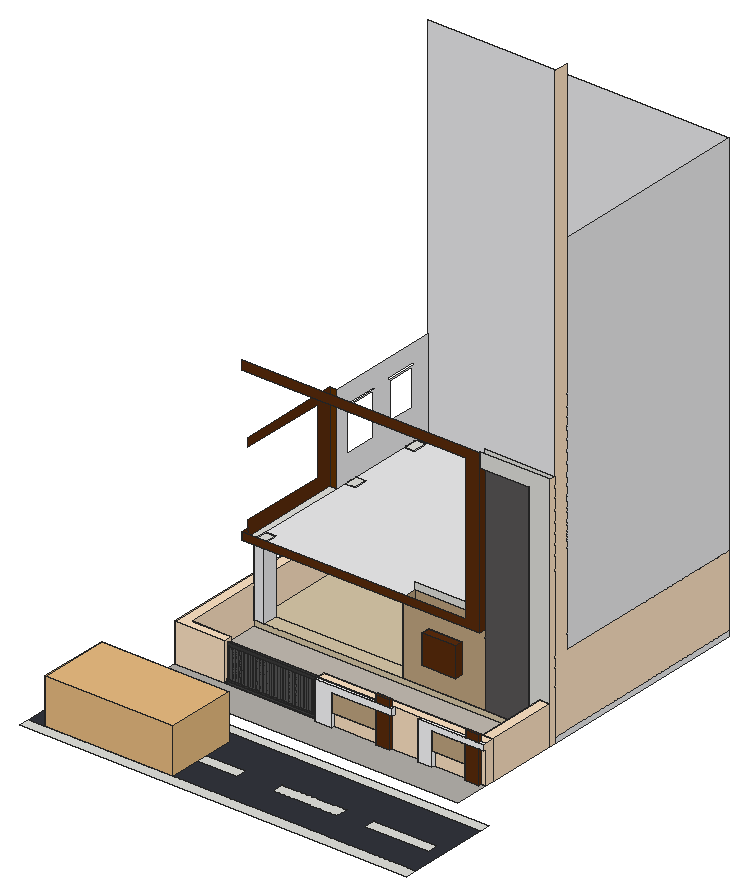
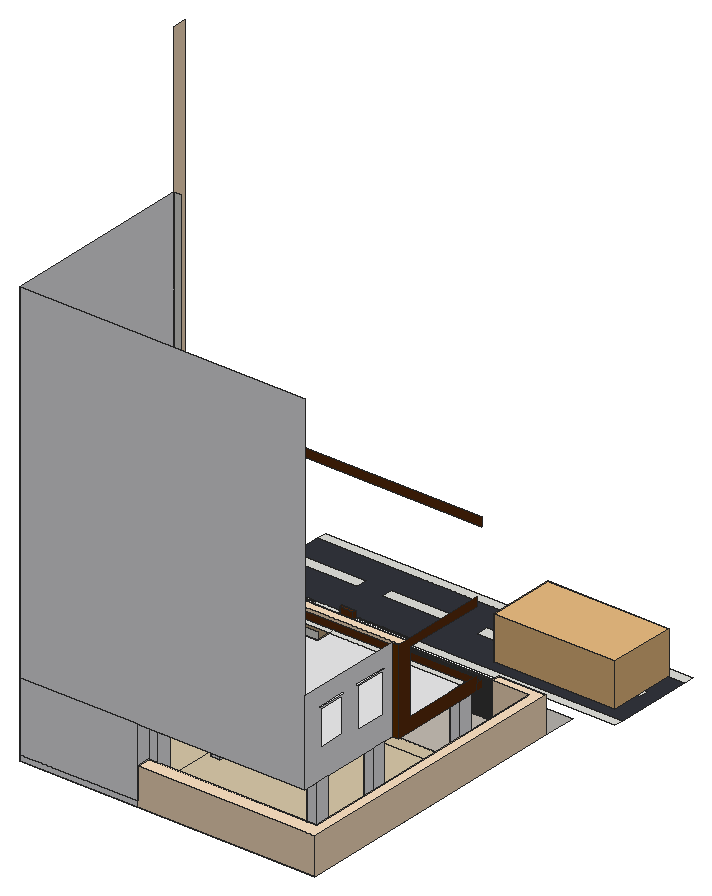
# SketchUp Ruby script. Lengths in inches.
U = 1.inch
M = Sketchup.active_model
def pt(a) = Geom::Point3d.new(a.map { |v| v * U })
def face(e, loops, mat)
  f = e.add_face(loops[0].map { |a| pt(a) })
  loops[1..].each { |l| e.add_face(l.map { |a| pt(a) }).erase! }
  f.material = f.back_material = mat if mat
  f
end
# faces: each face lists its corners as indices into pts; further lists are holes
def faces(e, pts, list, mat = nil) = list.each { |f| face(e, (f[0].is_a?(Array) ? f : [f]).map { |l| l.map { |i| pts[i] } }, mat) }
# xy, xz, yz: faces in a plane at the given z, y or x. An outline is a flat list of corners, or four numbers for a rectangle; further outlines are holes
def ring(l) = l.size == 4 ? [[l[0], l[1]], [l[2], l[1]], [l[2], l[3]], [l[0], l[3]]] : l.each_slice(2).to_a
def flat(e, list, mat, &to3) = list.each { |f| face(e, (f[0].is_a?(Array) ? f : [f]).map { |l| ring(l).map { |u, v| to3.(u, v) } }, mat) }
def xy(e, z, list, mat = nil) = flat(e, list, mat) { |x, y| [x, y, z] }
def xz(e, y, list, mat = nil) = flat(e, list, mat) { |x, z| [x, y, z] }
def yz(e, x, list, mat = nil) = flat(e, list, mat) { |y, z| [x, y, z] }
def lines(e, pts, list) = list.each { |a, b| e.add_line(pt(pts[a]), pt(pts[b])) }
# prism: a flat outline (further loops are holes) pulled along v
def prism(e, loops, v, mat = nil)
  f = face(e, loops, mat); d = Geom::Vector3d.new(v.map { |x| x * U })
  f.pushpull(f.normal.samedirection?(d) ? d.length : -d.length)
end
def box(e, o, s, mat = nil) = prism(e, [[o, [o[0] + s[0], o[1], o[2]], [o[0] + s[0], o[1] + s[1], o[2]], [o[0], o[1] + s[1], o[2]]]], [0, 0, s[2]], mat)
def at(x, y, z, deg = 0) = Geom::Transformation.translation(pt([x, y, z])) * Geom::Transformation.rotation(ORIGIN, Z_AXIS, deg.degrees)
def axes(o, x, y, z) = Geom::Transformation.new([*x, 0, *y, 0, *z, 0, *pt(o).to_a, 1])
def part(name) = M.definitions.add(name)
# library, detail: a bought-in or finely detailed component or shape, given as its bounding box
def library(name, o, s) = part(name).tap { |d| box(d.entities, o, s) }
def detail(e, o, s) = box(e.add_group.entities, o, s)
def put(e, d, t, mat = nil) = e.add_instance(d, t).tap { |i| i.material = mat if mat }
def group(e, t, mat = nil) = e.add_group.tap { |g| g.transformation = t; g.material = mat if mat }.entities
root = M.entities
M.materials.add("[0012_Bisque]").color = [255, 228, 196]
M.materials.add("[0035_Tan]").color = [188, 161, 125]
M.materials.add("[0035_Tan]1").color = [193, 166, 129]
M.materials.add("[0043_SaddleBrown]").color = [91, 44, 12]
M.materials.add("[Blinds Vertical Pattern]").color = [237, 237, 239]
M.materials.add("[Brick Tumbled]").color = [89, 87, 87]
M.materials.add("[Color C08]").color = [102, 51, 0]
M.materials.add("[Color M06]").color = [86, 86, 86]
M.materials.add("[Color M07]").color = [58, 58, 58]
M.materials.add("[Field Rectangle Tile]").color = [196, 189, 179]
M.materials.add("[Field Square Tile]").color = [217, 201, 169]
M.materials.add("[Formica Laminate Dark]1").color = [50, 53, 60]
M.materials.add("[Quartz Light Grey]").color = [251, 251, 252]
M.materials.add("[Tile Travertine 2 inch]").color = [181, 178, 172]
c1 = library("skpE847",[-111.76,-15.01,0.76],[2.12,4.6,1.82])
c2 = part("car+1")
p = [[0,0,0],[1,0,0],[1,1,0]]
lines(c2.entities,p,[[0,1],[1,2],[2,0]])
put(c2.entities,c1,axes([-477.97,5140.8,-31.25],[0,46,0],[-46,0,0],[0,0,40.94]))
xy(root,0,[[0,0,641.75,17.59],[22.28,68.03,129.53,88.03],[198.41,68.03,305.66,88.03],[364.41,68.03,471.66,88.03],[516.03,68.03,623.28,88.03],
  [0,153.78,641.75,169.75],[537.68,383.84,572.32,393.34],[56.22,393.34,572.32,753.91]])
xy(root,0,[[73.92,264.9,73.92,393.34,537.68,393.34,537.68,383.84,555.09,383.84,555.09,264.9]],"[Field Rectangle Tile]")
xy(root,0,[[[0,17.59,641.75,153.78],[516.03,68.03,623.28,88.03],[364.41,68.03,471.66,88.03],[198.41,68.03,305.66,88.03],[22.28,68.03,129.53,88.03]]],"[Formica Laminate Dark]1")
xy(root,0,[[292.71,246.01,320.3125,250.82],[392.59,246.01,416.02,250.82],[463.56,246.01,486.63,250.82],[541.28,246.01,564.49,250.82],[56.22,250.82,56.22,393.34,73.92,393.34,73.92,264.9,138.4,264.9,138.4,250.82],
  [138.4,250.82,292.71,264.9],[292.71,250.82,572.32,264.9],[555.09,264.9,572.32,383.84]],"[Quartz Light Grey]")
xy(root,0,[[56.22,192.09,56.22,250.82,292.71,250.82,292.71,246.01,320.3125,246.01,320.3125,250.82,392.59,250.82,392.59,246.01,416.02,246.01,416.02,250.82,463.56,250.82,463.56,246.01,486.63,246.01,486.63,250.82,541.28,250.82,541.28,246.01,564.49,246.01,564.49,250.82,572.32,250.82,572.32,192.09]],"[Tile Travertine 2 inch]")
xy(root,1.375,[[138.4,250.82,292.71,255.91],[138.4,260.85,292.71,264.9]],"[Color M07]")
xy(root,4.375,[[141.84,255.91,289.65,260.85]],"[Quartz Light Grey]")
xy(root,9,[[73.92,393.34,90.37,416.85],[320.99,393.34,320.99,418.04,554.62,418.04,537.68,393.34],[537.68,393.34,554.62,418.04,554.62,729.22,366.77,729.22,366.77,753.91,572.32,753.91,572.32,393.34],[350.92,565.72,367.46,593.6875],[73.92,581.84,90.37,604.84],
  [350.92,703.53,367.46,729.22],[73.92,704.28,90.37,729.22]])
xy(root,9,[[90.37,393.34,320.99,418.04],[[73.92,416.85,90.37,416.85,90.37,418.04,375.47,418.04,375.47,729.22,367.46,729.22,367.46,703.53,350.92,703.53,350.92,729.22,90.37,729.22,90.37,704.28,73.92,704.28,73.92,604.84,90.37,604.84,90.37,581.84,73.92,581.84],[350.92,565.72,367.46,593.6875]],[375.47,418.04,554.62,729.22]],"[Field Square Tile]")
xy(root,22.8,[[320.3125,246.01,392.59,250.82]],"[0035_Tan]1")
xy(root,24.29,[[486.63,246.01,541.28,250.82]],"[0035_Tan]1")
xy(root,49.04,[[362.89,379.84,418.71,393.34]],"[0043_SaddleBrown]")
xy(root,52.25,[[320.3125,246.01,392.59,250.82],[392.59,246.01,416.02,250.82],[416.02,246.01,420.375,250.82]],"[Quartz Light Grey]")
xy(root,53.97,[[486.63,246.01,541.28,250.82],[541.28,246.01,564.49,250.82],[564.49,246.01,572.32,250.82]],"[Quartz Light Grey]")
xy(root,58.9375,[[138.4,255.91,289.65,260.85],[289.65,255.91,292.71,260.85]],"[Color M07]")
xy(root,63.375,[[392.59,246.01,415.91,250.82],[542.59,246.01,564.49,250.82]])
xy(root,63.375,[[56.22,250.82,138.4,250.82,138.4,264.9,73.92,264.9,73.92,729.22,366.77,729.22,366.77,753.91,56.22,753.91],[292.71,250.82,572.32,264.9],[555.09,264.9,572.32,383.84]],"[0012_Bisque]")
xy(root,63.375,[[292.71,246.01,392.59,250.82],[415.91,246.01,420.375,250.82],[463.56,246.01,542.59,250.82],[564.49,246.01,572.32,250.82]],"[Quartz Light Grey]")
xy(root,74.9375,[[392.59,246.01,415.91,250.82],[542.59,246.01,564.49,250.82]],"[0043_SaddleBrown]")
xy(root,97.35,[[362.89,379.84,418.71,393.34]],"[0043_SaddleBrown]")
xy(root,129,[[63.07,382.09,73.92,393.34],[73.92,382.09,90.37,393.34],[90.37,382.09,320.99,393.34],[320.99,382.09,456.39,393.34],[63.07,393.34,73.92,564.01],
  [73.92,393.34,90.37,416.85],[554.62,418.04,572.32,753.91],[350.92,565.72,367.46,593.6875],[73.92,581.84,90.37,604.84],[350.92,703.53,367.46,729.22],
  [73.92,704.28,90.37,729.22],[73.92,729.22,90.37,753.91],[350.92,729.22,366.77,753.91],[366.77,729.22,367.46,753.91],[367.46,729.22,375.47,753.91],
  [375.47,729.22,554.62,753.91]])
xy(root,129,[[[90.37,393.34,90.37,416.85,73.92,416.85,73.92,581.84,90.37,581.84,90.37,604.84,73.92,604.84,73.92,704.28,90.37,704.28,90.37,753.91,350.92,753.91,350.92,703.53,367.46,703.53,367.46,729.22,554.62,729.22,554.62,418.04,320.99,418.04,320.99,393.34],[350.92,565.72,367.46,593.6875]]],"[Blinds Vertical Pattern]")
xz(root,246.01,[[320.3125,22.8,392.59,52.25],[486.63,24.29,541.28,53.97]],"[0035_Tan]1")
xz(root,246.01,[[392.59,0,416.02,52.25],[541.28,0,564.49,53.97],[392.59,63.375,415.91,74.9375],[542.59,63.375,564.49,74.9375]],"[0043_SaddleBrown]")
xz(root,246.01,[[292.71,0,320.3125,0,320.3125,52.25,420.375,52.25,420.375,63.375,292.71,63.375],[463.56,0,486.63,0,486.63,53.97,572.32,53.97,572.32,63.375,463.56,63.375]],"[Quartz Light Grey]")
xz(root,250.82,[[56.22,0,138.4,63.375],[320.3125,0,392.59,22.8],[416.02,0,463.56,0,463.56,63.375,420.375,63.375,420.375,52.25,416.02,52.25],[486.63,0,541.28,24.29],[564.49,0,572.32,53.97]],"[0012_Bisque]")
xz(root,250.82,[[392.59,63.375,415.91,74.9375],[542.59,63.375,564.49,74.9375]],"[0043_SaddleBrown]")
xz(root,250.82,[[138.4,0,292.71,1.375]],"[Color M07]")
xz(root,250.82,[[292.71,0,292.71,63.375,420.375,63.375,420.375,52.25,320.3125,52.25,320.3125,0],[392.59,0,416.02,52.25],[541.28,0,564.49,53.97],[320.3125,22.8,392.59,52.25],[486.63,24.29,541.28,53.97]],"[Quartz Light Grey]")
xz(root,255.91,[[141.84,4.375,146.21,54.59],[146.21,4.375,148.04,54.59],[148.04,4.375,151.9,54.59],[151.9,4.375,153.73,54.59],[153.73,4.375,157.58,54.59],
  [157.58,4.375,159.41,54.59],[159.41,4.375,163.27,54.59],[163.27,4.375,165.1,54.59],[165.1,4.375,168.96,54.59],[168.96,4.375,170.79,54.59],
  [170.79,4.375,174.65,54.59],[174.65,4.375,176.48,54.59],[176.48,4.375,180.33,54.59],[180.33,4.375,182.16,54.59],[182.16,4.375,186.02,54.59],
  [186.02,4.375,187.85,54.59],[187.85,4.375,191.71,54.59],[191.71,4.375,193.54,54.59],[193.54,4.375,197.4,54.59],[197.4,4.375,199.23,54.59],
  [199.23,4.375,203.08,54.59],[203.08,4.375,204.91,54.59],[204.91,4.375,209.15,54.59],[209.15,4.375,210.98,54.59],[210.98,4.375,215.21,54.59],
  [215.21,4.375,217.04,54.59],[217.04,4.375,221.27,54.59],[221.27,4.375,223.1,54.59],[223.1,4.375,227.33,54.59],[227.33,4.375,229.16,54.59],
  [229.16,4.375,233.4,54.59],[233.4,4.375,235.23,54.59],[235.23,4.375,239.46,54.59],[239.46,4.375,241.29,54.59],[241.29,4.375,245.52,54.59],
  [245.52,4.375,247.35,54.59],[247.35,4.375,251.58,54.59],[251.58,4.375,253.41,54.59],[253.41,4.375,257.9,54.59],[257.9,4.375,259.73,54.59],
  [259.73,4.375,264.33,54.59],[264.33,4.375,266.16,54.59],[266.16,4.375,270.77,54.59],[270.77,4.375,272.6,54.59],[272.6,4.375,277.02,54.59],
  [277.02,4.375,278.85,54.59],[278.85,4.375,282.42,54.59],[282.42,4.375,284.25,54.59],[284.25,4.375,289.65,54.59]],"[Color M06]")
xz(root,255.91,[[[138.4,1.375,292.71,58.9375],[141.84,4.375,289.65,54.59]]],"[Color M07]")
xz(root,260.85,[[138.4,1.375,292.71,4.375],[138.4,4.375,138.4,58.9375,289.65,58.9375,289.65,54.59,141.84,54.59,141.84,4.375],[141.84,4.375,289.65,54.59],[289.65,4.375,292.71,58.9375]],"[Color M07]")
xz(root,264.9,[[73.92,0,138.4,63.375],[292.71,0,555.09,63.375]],"[0012_Bisque]")
xz(root,264.9,[[138.4,0,146.67,1.375],[146.67,0,292.71,1.375],[555.09,0,572.32,63.375]],"[Quartz Light Grey]")
xz(root,379.84,[[362.89,49.04,418.71,97.35]],"[0043_SaddleBrown]")
xz(root,382.09,[[63.07,129,456.39,129,456.39,397.0625,63.07,397.0625,63.07,381.625,434.25,381.625,434.25,141.625,63.07,141.625]],"[0043_SaddleBrown]")
xz(root,383.84,[[537.68,0,555.09,0,555.09,63.375,572.32,63.375,572.32,397.0625,456.39,397.0625,456.39,373.6,537.68,373.6]])
xz(root,383.84,[[555.09,0,572.32,63.375]],"[Quartz Light Grey]")
xz(root,393.34,[[537.68,0,572.32,9],[537.68,9,537.68,373.6,456.39,373.6,456.39,397.0625,572.32,397.0625,572.32,9],[362.89,49.04,418.71,97.35]])
xz(root,393.34,[[[320.99,9,456.39,129],[362.89,49.04,418.71,97.35]]],"[0035_Tan]1")
xz(root,393.34,[[73.92,9,90.37,129]],"[Blinds Vertical Pattern]")
xz(root,393.34,[[456.39,9,537.68,373.6]],"[Brick Tumbled]")
xz(root,393.34,[[73.92,0,537.68,9]],"[Field Square Tile]")
xz(root,416.85,[[73.92,9,90.37,129]],"[Blinds Vertical Pattern]")
xz(root,418.04,[[320.99,129,554.62,141.625],[554.62,129,572.32,129,572.32,741.625,560.26,741.625,560.26,141.625,554.62,141.625]])
xz(root,418.04,[[320.99,9,554.62,129]],"[0035_Tan]")
xz(root,564.01,[[63.07,129,73.92,276.4375]],"[Color C08]")
xz(root,565.72,[[350.92,9,367.46,129]],"[Blinds Vertical Pattern]")
xz(root,581.84,[[73.92,9,90.37,129]],"[Blinds Vertical Pattern]")
xz(root,593.6875,[[350.92,9,367.46,129]],"[Blinds Vertical Pattern]")
xz(root,604.84,[[73.92,9,90.37,129]],"[Blinds Vertical Pattern]")
xz(root,703.53,[[350.92,9,367.46,129]],"[Blinds Vertical Pattern]")
xz(root,704.28,[[73.92,9,90.37,129]],"[Blinds Vertical Pattern]")
xz(root,729.22,[[73.92,9,90.37,63.375],[350.92,9,366.77,63.375],[366.77,9,367.46,129]])
xz(root,729.22,[[90.37,9,350.92,63.375]],"[0012_Bisque]")
xz(root,729.22,[[367.46,9,554.62,129],[73.92,63.375,90.37,129],[350.92,63.375,366.77,129]],"[Blinds Vertical Pattern]")
xz(root,753.91,[[56.22,0,366.77,63.375]],"[0012_Bisque]")
xz(root,753.91,[[366.77,0,572.32,9],[366.77,9,572.32,129],[73.92,129,572.32,741.625]],"[Blinds Vertical Pattern]")
yz(root,56.22,[[250.82,0,753.91,63.375]],"[0012_Bisque]")
yz(root,63.07,[[382.09,129,393.34,141.625],[393.34,129,393.34,153.1875,538.2,153.1875,538.2,261.625,393.34,261.625,393.34,276.4375,564.01,276.4375,564.01,129]],"[0043_SaddleBrown]")
yz(root,73.92,[[393.34,9,416.85,63.375],[581.84,9,604.84,63.375],[704.28,9,729.22,63.375]])
yz(root,73.92,[[264.9,0,393.34,63.375],[416.85,9,581.84,63.375],[604.84,9,704.28,63.375]],"[0012_Bisque]")
yz(root,73.92,[[393.34,63.375,416.85,129],[581.84,63.375,604.84,129],[704.28,63.375,729.22,129],[[564.01,129,753.91,276.4375],[584.76,172.06,639.13,241.06],[674.3125,181.06,720.75,241.56],[580.82,242.21,643.76,246.02],[669.92,243.04,724.48,246.66]]],"[Blinds Vertical Pattern]")
yz(root,90.37,[[393.34,9,416.85,129],[581.84,9,604.84,129],[704.28,9,729.22,129]],"[Blinds Vertical Pattern]")
yz(root,138.4,[[250.82,1.375,255.91,1.375,255.91,58.9375,260.85,58.9375,260.85,1.375,264.9,1.375,264.9,63.375,250.82,63.375]],"[0012_Bisque]")
yz(root,138.4,[[250.82,0,264.9,0,264.9,1.375,260.85,1.375,260.85,4.375,255.91,4.375,255.91,1.375,250.82,1.375],[255.91,4.375,260.85,58.9375]],"[Quartz Light Grey]")
yz(root,141.84,[[255.91,4.375,260.85,54.59]],"[Quartz Light Grey]")
yz(root,289.65,[[255.91,4.375,260.85,54.59]],"[Quartz Light Grey]")
yz(root,292.71,[[250.82,1.375,250.82,63.375,264.9,63.375,264.9,1.375,260.85,1.375,260.85,58.9375,255.91,58.9375,255.91,1.375]],"[0012_Bisque]")
yz(root,292.71,[[246.01,0,250.82,63.375],[250.82,0,250.82,1.375,255.91,1.375,255.91,4.375,260.85,4.375,260.85,1.375,264.9,1.375,264.9,0],[255.91,4.375,260.85,58.9375]],"[Quartz Light Grey]")
yz(root,320.3125,[[246.01,0,250.82,22.8],[246.01,22.8,250.82,52.25]],"[Quartz Light Grey]")
yz(root,320.99,[[393.34,9,418.04,129]],"[0035_Tan]")
yz(root,350.92,[[565.72,9,593.6875,129],[703.53,9,729.22,129]],"[Blinds Vertical Pattern]")
yz(root,362.89,[[379.84,49.04,393.34,97.35]],"[0043_SaddleBrown]")
yz(root,366.77,[[729.22,9,753.91,63.375]])
yz(root,366.77,[[729.22,63.375,753.91,129]],"[Blinds Vertical Pattern]")
yz(root,367.46,[[565.72,9,593.6875,129],[703.53,9,729.22,129]],"[Blinds Vertical Pattern]")
yz(root,392.59,[[246.01,0,250.82,22.8],[246.01,63.375,250.82,74.9375]],"[0043_SaddleBrown]")
yz(root,392.59,[[246.01,22.8,250.82,52.25]],"[Quartz Light Grey]")
yz(root,415.91,[[246.01,63.375,250.82,74.9375]],"[0043_SaddleBrown]")
yz(root,416.02,[[246.01,0,250.82,52.25]],"[0043_SaddleBrown]")
yz(root,418.71,[[379.84,49.04,393.34,97.35]],"[0043_SaddleBrown]")
yz(root,420.375,[[246.01,52.25,250.82,63.375]],"[Quartz Light Grey]")
yz(root,456.39,[[382.09,129,393.34,129,393.34,373.6,383.84,373.6,383.84,397.0625,382.09,397.0625]],"[0043_SaddleBrown]")
yz(root,463.56,[[246.01,0,250.82,63.375]],"[Quartz Light Grey]")
yz(root,486.63,[[246.01,0,250.82,24.29],[246.01,24.29,250.82,53.97]],"[Quartz Light Grey]")
yz(root,537.68,[[383.84,0,393.34,373.6]])
yz(root,541.28,[[246.01,0,250.82,24.29]],"[0043_SaddleBrown]")
yz(root,541.28,[[246.01,24.29,250.82,53.97]],"[Quartz Light Grey]")
yz(root,542.59,[[246.01,63.375,250.82,74.9375]],"[0043_SaddleBrown]")
yz(root,554.62,[[418.04,9,729.22,129]],"[Blinds Vertical Pattern]")
yz(root,555.09,[[264.9,0,383.84,63.375]],"[0012_Bisque]")
yz(root,564.49,[[246.01,0,250.82,53.97],[246.01,63.375,250.82,74.9375]],"[0043_SaddleBrown]")
yz(root,572.32,[[250.82,0,264.9,0,264.9,63.375,246.01,63.375,246.01,53.97,250.82,53.97],[264.9,0,383.84,63.375],[383.84,0,393.34,397.0625],[393.34,9,753.91,9,753.91,129,418.04,129,418.04,999.875,393.34,999.875]],"[0012_Bisque]")
yz(root,572.32,[[393.34,0,753.91,9],[418.04,129,753.91,741.625]],"[Blinds Vertical Pattern]")
p = [[73.92,538.2,141.625],[73.92,538.2,129]]
lines(root,p,[[0,1]])
put(root,c2,axes([27.1,17.59,0],[1,0,0],[0,1.2,0],[0,0,1]))
